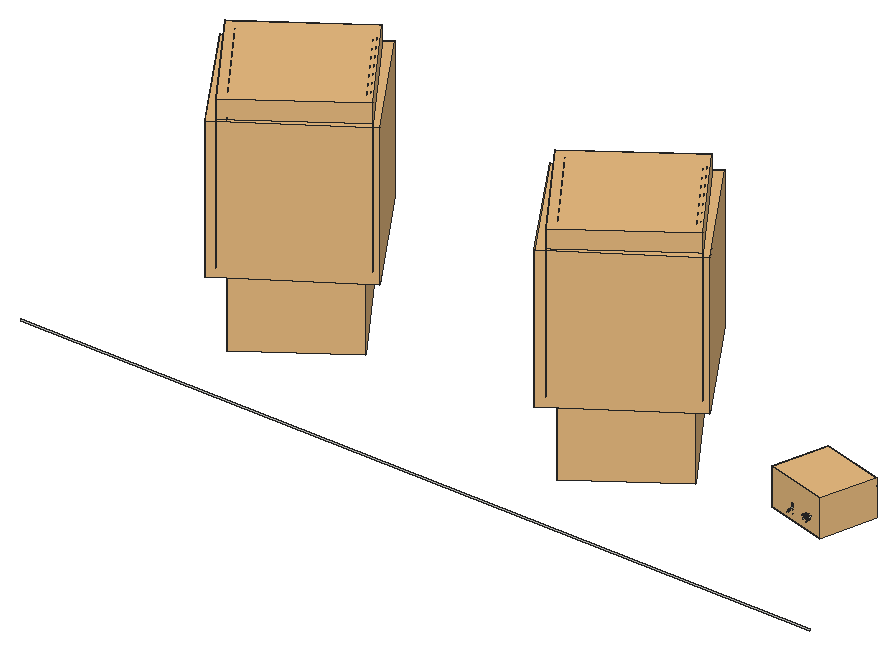
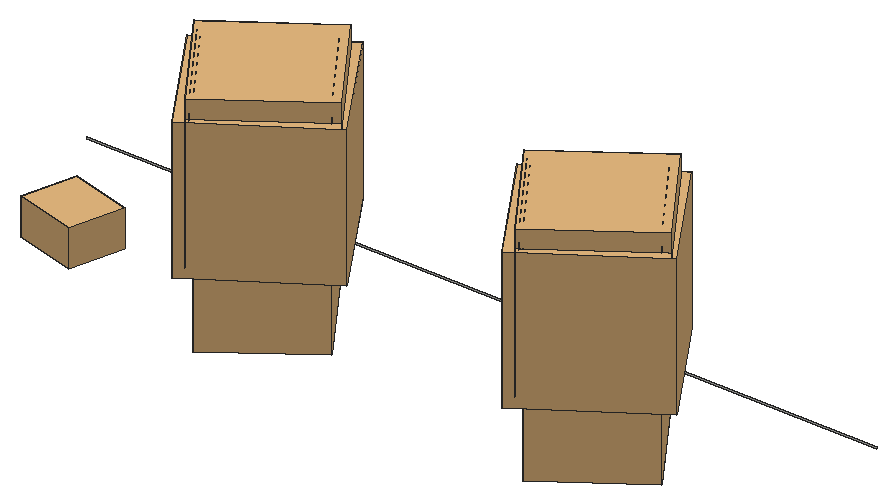
# SketchUp Ruby script. Lengths in inches.
U = 1.inch
M = Sketchup.active_model
def pt(a) = Geom::Point3d.new(a.map { |v| v * U })
def face(e, loops, mat)
  f = e.add_face(loops[0].map { |a| pt(a) })
  loops[1..].each { |l| e.add_face(l.map { |a| pt(a) }).erase! }
  f.material = f.back_material = mat if mat
  f
end
# faces: each face lists its corners as indices into pts; further lists are holes
def faces(e, pts, list, mat = nil) = list.each { |f| face(e, (f[0].is_a?(Array) ? f : [f]).map { |l| l.map { |i| pts[i] } }, mat) }
# xy, xz, yz: faces in a plane at the given z, y or x. An outline is a flat list of corners, or four numbers for a rectangle; further outlines are holes
def ring(l) = l.size == 4 ? [[l[0], l[1]], [l[2], l[1]], [l[2], l[3]], [l[0], l[3]]] : l.each_slice(2).to_a
def flat(e, list, mat, &to3) = list.each { |f| face(e, (f[0].is_a?(Array) ? f : [f]).map { |l| ring(l).map { |u, v| to3.(u, v) } }, mat) }
def xy(e, z, list, mat = nil) = flat(e, list, mat) { |x, y| [x, y, z] }
def xz(e, y, list, mat = nil) = flat(e, list, mat) { |x, z| [x, y, z] }
def yz(e, x, list, mat = nil) = flat(e, list, mat) { |y, z| [x, y, z] }
def lines(e, pts, list) = list.each { |a, b| e.add_line(pt(pts[a]), pt(pts[b])) }
# prism: a flat outline (further loops are holes) pulled along v
def prism(e, loops, v, mat = nil)
  f = face(e, loops, mat); d = Geom::Vector3d.new(v.map { |x| x * U })
  f.pushpull(f.normal.samedirection?(d) ? d.length : -d.length)
end
def box(e, o, s, mat = nil) = prism(e, [[o, [o[0] + s[0], o[1], o[2]], [o[0] + s[0], o[1] + s[1], o[2]], [o[0], o[1] + s[1], o[2]]]], [0, 0, s[2]], mat)
def at(x, y, z, deg = 0) = Geom::Transformation.translation(pt([x, y, z])) * Geom::Transformation.rotation(ORIGIN, Z_AXIS, deg.degrees)
def axes(o, x, y, z) = Geom::Transformation.new([*x, 0, *y, 0, *z, 0, *pt(o).to_a, 1])
def part(name) = M.definitions.add(name)
# library, detail: a bought-in or finely detailed component or shape, given as its bounding box
def library(name, o, s) = part(name).tap { |d| box(d.entities, o, s) }
def detail(e, o, s) = box(e.add_group.entities, o, s)
def put(e, d, t, mat = nil) = e.add_instance(d, t).tap { |i| i.material = mat if mat }
def group(e, t, mat = nil) = e.add_group.tap { |g| g.transformation = t; g.material = mat if mat }.entities
root = M.entities
M.materials.add("028_190k_fullGeometry_Material \#4").color = [120, 148, 64]
M.materials.add("0ad16as01f6asdLeafVar1sfd015as60f1as6").color = [231, 235, 211]
M.materials.add("asdfasdf0165f6asdLeafVar1sfd015as60f1as6").color = [231, 235, 211]
M.materials.add("dw_stemssadfasdfa0sdf1s01d6w1").color = [90, 97, 50]
c1 = library("028_190k_fullGeometry_0",[-319.99,-281.1,-2.15],[577.33,562.38,1159.36])
c2 = library("028_190k_fullGeometry_1",[-333.4,-281.7,421.48],[600.33,578.53,738.83])
c3 = library("028_190k_fullGeometry_2",[-3584003,-3264710,4041818.25],[6566285.5,6460741.75,7903602.75])
c4 = library("028_190k_fullGeometry_3",[-353.86,-324.57,405.22],[652.24,636.69,781.83])
c5 = part("028_190k_fullGeometry_4")
p = [[125.51,152.8,882.93],[125.36,152.82,883.01],[124.8,155.5625,881.05]]
faces(c5.entities,p,[[0,1,2]],"028_190k_fullGeometry_Material \#4")
c6 = part("028_190k_fullGeometry")
g1 = group(c6.entities,at(0,0,0))
put(g1,c1,axes([0,0,0],[0.18998,-0.26642,0],[0.26642,0.18998,0],[0,0,0.32722]))
put(g1,c2,axes([0,0,0],[0.18998,-0.26642,0],[0.26642,0.18998,0],[0,0,0.32722]))
put(g1,c3,axes([0,0,0],[0.00002,-0.00003,0],[0.00003,0.00002,0],[0,0,0.00003]))
put(g1,c4,axes([0,0,0],[0.18998,-0.26642,0],[0.26642,0.18998,0],[0,0,0.32722]))
put(g1,c5,axes([0,0,0],[0.18998,-0.26642,0],[0.26642,0.18998,0],[0,0,0.32722]))
c7 = part("vdw_leaf\#3")
p = [[0,0,0],[-2.77,1.61,2.32],[-4.3125,6.1,4.5],[-3.97,13.49,6.09],[-2.47,18.57,6.3],[-0.2,22.73,5.75],
  [2.54,19.66,6.85],[4.3,15.93,7.09],[5.03,7.6,5.43],[3.32,1.76,2.74]]
faces(c7.entities,p,[[0,1,2,3,4,5],[0,5,6,7,8,9]],"asdfasdf0165f6asdLeafVar1sfd015as60f1as6")
c8 = part("dw_brancj_2\#2")
p = [[9.7,-0.22,29.95],[0.23,-1.96,0.34],[-0.05,1.51,0.11],[9.65,1.51,29.46],[18.64,-8.75,84.43],[18.96,-6.63,84.625],
  [1.53,6.02,63.68],[1.42,8.18,63.25],[-10.58,8.77,161.17],[-10.41,9.98,160.68],[26.34,-9.37,211.72],[26.57,-8.28,211.23]]
faces(c8.entities,p,[[0,1,2],[0,2,3],[4,0,3],[4,3,5],[6,0,3],[6,3,7],[8,6,7],[8,7,9],
  [10,4,5],[10,5,11]],"dw_stemssadfasdfa0sdf1s01d6w1")
c9 = part("vdw_branch2\#3")
put(c9.entities,c7,axes([19.53,-5.9,102.42],[1.12377,-0.50004,0],[0.46097,1.03596,0.47664],[-0.19377,-0.43548,1.13389]))
put(c9.entities,c7,axes([-5.89,6.52,109.44],[-1.07209,0.83679,0],[-0.77141,-0.98832,0.52702],[0.32427,0.41545,1.25373]))
put(c9.entities,c7,axes([-0.44,8.23,75.28],[0.88709,-0.9947,0],[0.92159,0.82189,0.33087],[-0.25219,-0.22491,1.26111]))
put(c9.entities,c7,axes([24.71,-8.97,190.81],[-0.82641,0.91101,0],[-0.83983,-0.76184,0.47664],[0.35303,0.32025,1.13389]))
put(c9.entities,c7,axes([-2.29,8.24,91.35],[1.24603,-0.47303,0],[0.43826,1.15445,0.33087],[-0.11993,-0.31592,1.26111]))
put(c9.entities,c7,axes([12.26,-3.11,37.92],[-0.64625,1.02205,0.22511],[-1.04383,-0.61044,-0.22511],[-0.07533,-0.30931,1.18809]))
put(c9.entities,c7,axes([26.17,-9.17,210.27],[-0.99452,-0.10453,0],[0.09636,-0.91681,0.38752],[-0.04051,0.38539,0.92186]))
put(c9.entities,c7,axes([-6.07,9.4,125.35],[-0.90214,-0.98107,0],[0.90896,-0.83583,0.33087],[-0.24874,0.22873,1.26111]))
put(c9.entities,c7,axes([-4.13,7.29,110.58],[0.44715,-1.078,0.64369],[1.05816,0.63649,0.33087],[-0.58725,0.40856,1.09216]))
put(c9.entities,c7,axes([23.91,-8.22,171.96],[0.62307,0.85009,-0.63406],[-0.71531,0.8798,0.47664],[0.78296,0.12729,0.94004]))
put(c9.entities,c8,at(-0.09,0.18,-0.25),"dw_stemssadfasdfa0sdf1s01d6w1")
put(c9.entities,c7,axes([23.34,-9.65,156.59],[-0.31364,-1.00782,0.58216],[1.10369,-0.17062,0.29925],[-0.17137,0.6239,0.98776]))
put(c9.entities,c7,axes([15.03,-3.37,58.83],[-1.05425,-0.00194,0.58442],[-0.14303,-1.11707,-0.26172],[0.55355,-0.3046,0.99755]))
put(c9.entities,c7,axes([-11.625,9.46,160.37],[0.36812,0.92978,0],[-0.85713,0.33936,0.38752],[0.3603,-0.14265,0.92186]))
put(c9.entities,c7,axes([21.32,-8.53,138.72],[1.21379,0.19904,0],[-0.19904,1.21379,0],[0,0,1.23]))
put(c9.entities,c7,axes([22.54,-9.2,141.43],[-1.02887,0.17955,0.60182],[-0.23387,-1.13057,-0.06253],[0.56696,-0.17376,1.02111]))
put(c9.entities,c7,axes([23.9,-8.82,173.84],[-1.14567,-0.37474,0],[0.35918,-1.0981,0.04438],[-0.01409,0.04308,1.17993]))
put(c9.entities,c7,axes([-7.84,8.92,143.59],[-1.26971,0.40522,0],[-0.37543,-1.17638,0.33087],[0.10274,0.32192,1.26111]))
put(c9.entities,c7,axes([19.77,-8.01,85.98],[-0.32405,-1.14591,0.18674],[1.10278,-0.32969,-0.10948],[0.15845,0.14442,1.16117]))
put(c9.entities,c7,axes([-0.62,5.76,76.34],[-0.08879,1.17576,-0.67771],[-1.34525,-0.16582,-0.11144],[-0.17897,0.66309,1.17383]))
put(c9.entities,c7,axes([20.49,-8.22,121.07],[0.39924,-0.78471,-0.8233],[1.08735,0.33121,0.2116],[0.09035,-0.83005,0.83495]))
put(c9.entities,c7,axes([15.15,-3.72,62.9],[1.16251,0.40128,-0.0211],[-0.39924,1.16074,0.07874],[0.0456,-0.06757,1.2273]))
put(c9.entities,c7,axes([20.72,-8.08,120.26],[-0.03693,1.2277,-0.06551],[-1.22944,-0.03698,0],[-0.00197,0.06548,1.22825]))
put(c9.entities,c7,axes([22.58,-8.36,155.57],[-0.56247,1.09386,0],[-1.00839,-0.51852,0.47664],[0.42389,0.21796,1.13389]))
put(c9.entities,c7,axes([3.97,3.13,57.96],[-1.09459,0.76041,0],[-0.72262,-1.0402,-0.1735],[-0.10109,-0.14552,1.29352]))
put(c9.entities,c7,axes([-10.8,9.06,160.75],[-0.66334,-0.72138,0],[0.66835,-0.61458,0.24329],[-0.1829,0.16818,0.92729]))
put(c9.entities,c7,axes([19.06,-9.3125,103.96],[-1.01345,0.25553,-0.60051],[-0.2265,-1.12952,-0.09839],[-0.59598,0.03076,1.01889]))
put(c9.entities,c7,axes([18.07,-6.2,81.7],[-0.56247,1.09386,0],[-1.00839,-0.51852,0.47664],[0.42389,0.21796,1.13389]))
put(c9.entities,c7,axes([12.95,-0.39,43.31],[0.13044,-1.19832,0],[1.11025,0.12085,0.29925],[-0.30382,-0.03307,1.14057]))
put(c9.entities,c7,axes([2.28,8.28,56.18],[1.32413,-0.31027,0],[0.30923,1.31968,-0.11144],[0.02542,0.1085,1.35543]))
put(c9.entities,c7,axes([-7.55,9.96,143.07],[1.34251,-0.21744,0],[0.20045,1.23761,0.52702],[-0.08426,-0.52024,1.25373]))
put(c9.entities,c7,axes([26.15,-8.25,210.66],[0.94661,-0.25364,0],[0.235,0.87703,0.24329],[-0.06431,-0.24,0.92729]))
put(c9.entities,c7,axes([-6.48,11.37,125.16],[0.64635,1.10315,0.46356],[-1.16569,0.46153,0.52702],[0.27017,-0.6478,1.16488]))
put(c9.entities,c7,axes([25.74,-8.35,191.28],[0.13044,-1.19832,0],[1.11025,0.12085,0.29925],[-0.30382,-0.03307,1.14057]))
put(c9.entities,c7,axes([-5.125,7.47,91.6],[-1.10024,0.63688,0.48318],[-0.78682,-1.00808,-0.46292],[0.14137,-0.65404,1.184]))
c10 = part("vdw_leaf\#1")
p = [[0,0,0],[-2.77,1.61,2.32],[-4.3125,6.1,4.5],[-3.97,13.49,6.09],[-2.47,18.57,6.3],[-0.2,22.73,5.75],
  [2.54,19.66,6.85],[4.3,15.93,7.09],[5.03,7.6,5.43],[3.32,1.76,2.74]]
faces(c10.entities,p,[[0,1,2,3,4,5],[0,5,6,7,8,9]],"0ad16as01f6asdLeafVar1sfd015as60f1as6")
c11 = part("dw_branch_3\#2")
p = [[-10.06,-1.6,62.9],[-0.2,1.54,-0.01],[-10.43,1.54,62.72],[0.18,-1.6,0.17],[-23.75,-21.66,88.91],[-25.7,-20.3,89.55],
  [13.4,11.62,104.56],[13.33,13.52,104.47],[-49.25,-41.87,130.3125],[-50.33,-40.21,130.71],[-4.97,21.13,143.98],[35.61,27.99,178.64],
  [-5.09,23.64,143.96],[35.32,29.14,178.46],[-67.7,-55.38,181.06],[-68.34,-54.45,181.62],[-22.8125,33.9,200.59],[-22.94,35.79,200.41],
  [56.61,36.78,229.75],[56.29,38.09,229.57],[-70.63,-67.46,248.85],[-70.72,-66.33,249.5],[-25.05,43.32,240.75],[-24.98,44.26,240.57]]
faces(c11.entities,p,[[0,1,2],[0,3,1],[4,2,5],[4,0,2],[6,0,2],[6,2,7],[8,4,5],[8,5,9],
  [10,6,7],[11,6,7],[10,7,12],[11,7,13],[14,8,9],[14,9,15],[16,10,12],[16,12,17],
  [18,11,13],[18,13,19],[20,14,15],[20,15,21],[22,16,17],[22,17,23]],"dw_stemssadfasdfa0sdf1s01d6w1")
c12 = part("dw_branch3\#2")
put(c12.entities,c10,axes([-70.33,-63.58,233.32],[-1.00752,0.412,0.78596],[-0.24851,-1.22189,0.32195],[0.83141,0.09817,1.01433]))
put(c12.entities,c10,axes([-66.93,-54.91,182.82],[-0.84976,-0.98359,0.33619],[0.99572,-0.74889,0.32577],[-0.05223,0.46521,1.22907]))
put(c12.entities,c10,axes([-46.12,-39.49,126.35],[1.23843,0.5364,0.23552],[-0.56438,0.94474,0.81599],[0.15707,-0.83465,1.07498]))
put(c12.entities,c10,axes([13.0625,13.13,104.77],[-1.01271,0.69982,-0.26884],[-0.74268,-0.99813,0.19939],[-0.10222,0.31872,1.21473]))
put(c12.entities,c10,axes([-18.87,30.42,186.42],[0.36309,1.06515,-0.56675],[-1.14134,0.49515,0.19939],[0.39128,0.45593,1.10754]))
put(c12.entities,c10,axes([-3.2,4.15,75.77],[-1.04153,0.55414,0.44243],[-0.23365,-1.01045,0.71554],[0.6695,0.50943,0.93801]))
put(c12.entities,c10,axes([23.2,19.41,136.3],[-0.65687,-1.11295,-0.05714],[1.05857,-0.61429,-0.20411],[0.15163,-0.1536,1.24868]))
put(c12.entities,c10,axes([-25.57,35.48,201.32],[-0.64726,0.62827,0.87973],[-0.71635,-1.0172,0.19939],[0.80962,-0.39773,0.87973]))
put(c12.entities,c10,axes([-36.37,-32.14,110.35],[-0.80747,1.09962,0.12544],[-0.83333,-0.50188,-0.96467],[-0.72833,-0.64487,0.96467]))
put(c12.entities,c10,axes([-9.89,26.72,156.79],[0.45529,1.02969,0.56572],[-1.16919,0.33753,0.32662],[0.11537,-0.64297,1.07744]))
put(c12.entities,c10,axes([-26.57,46.1,241.0625],[0.00015,0.80921,0.22536],[-0.83985,0.00446,-0.01542],[-0.01605,-0.22532,0.80906]))
put(c12.entities,c10,axes([-9.2,-2.58,61.06],[-1.10001,-0.40312,0.39014],[0.40883,-1.1116,0.00411],[0.35732,0.13566,1.14763]))
put(c12.entities,c10,axes([-69.91,-63.11,233.93],[1.36249,-0.1432,0],[0.13201,1.25603,0.5309],[-0.05549,-0.52799,1.26295]))
put(c12.entities,c10,axes([32.2,25.46,166.13],[0.06878,-1.29051,-0.05714],[1.22165,0.07415,-0.20411],[0.2113,-0.04403,1.24868]))
put(c12.entities,c10,axes([-5.68,-0.66,44.43],[-0.48448,-1.12287,0.17078],[0.98138,-0.33653,0.57135],[-0.48308,0.36756,1.04626]))
put(c12.entities,c10,axes([43.45,32.81,198.64],[0.5408,1.19584,0.14106],[-0.94242,0.32409,0.86557],[0.74952,-0.45533,0.98656]))
put(c12.entities,c10,axes([12.52,14.14,104.98],[1.02694,0.54888,0.41092],[-0.53566,1.05407,-0.06927],[-0.38969,-0.12321,1.13846]))
put(c12.entities,c10,axes([44.55,32.375,198.73],[-0.65687,-1.11295,-0.05714],[1.05857,-0.61429,-0.20411],[0.15163,-0.1536,1.24868]))
put(c12.entities,c10,axes([-5.67,21.17,141.44],[-1.10726,0.43603,-0.32953],[-0.49537,-1.03435,0.29588],[-0.17521,0.40597,1.12589]))
put(c12.entities,c10,axes([55.69,37.84,229.48],[0.18984,0.96334,0.18958],[-0.71996,0.0053,0.69399],[0.66755,-0.26823,0.69457]))
put(c12.entities,c10,axes([-21.52,36.85,205.2],[0.72606,-0.98817,0.14519],[0.94364,0.7084,0.10251],[-0.16885,0.05176,1.19664]))
put(c12.entities,c10,axes([-68.51,-56.35,196.07],[1.16319,0.72381,0],[-0.66725,1.0723,0.5309],[0.28049,-0.45075,1.26295]))
put(c12.entities,c11,at(0.01,-0.09,-0.02),"dw_stemssadfasdfa0sdf1s01d6w1")
put(c12.entities,c10,axes([-2.49,5.18,75.91],[0.78614,-0.90346,-0.30078],[0.86953,0.79562,-0.11715],[0.28546,-0.14014,1.16705]))
put(c12.entities,c10,axes([-23.125,-16.22,82.25],[0.32175,1.32576,0.12544],[-1.33153,0.31835,0.05068],[0.01989,-0.13382,1.3633]))
put(c12.entities,c10,axes([-23.75,41.99,230.3],[0.85958,-0.87451,0.14519],[0.66531,0.75721,0.62192],[-0.54076,-0.36226,1.01955]))
put(c12.entities,c10,axes([27.07,22.48,149.34],[0.92952,-0.64745,-0.62467],[0.50188,1.074,-0.36637],[0.71693,0.02135,1.04468]))
put(c12.entities,c10,axes([17.66,16.25,119.93],[-0.91649,0.83891,-0.3601],[-0.87434,-0.77966,0.40896],[0.0492,0.54447,1.14321]))
put(c12.entities,c10,axes([-68.37,-54.54,181.63],[0.32047,1.28399,0.35434],[-1.33153,0.31835,0.05068],[-0.03484,-0.35624,1.32241]))
put(c12.entities,c10,axes([-28.98,-27.1,96.48],[-0.8814,-0.35966,-0.98523],[0.75246,-1.11336,-0.26672],[-0.73065,-0.71272,0.91382]))
put(c12.entities,c10,axes([-15.23,28.43,172.72],[-1.21149,0.11898,0.32517],[-0.09739,-1.25259,0.09551],[0.33228,0.0667,1.21356]))
put(c12.entities,c10,axes([-17.5625,31.23,186.85],[-0.49275,-1.12287,0.14519],[0.95014,-0.33653,0.62192],[-0.53717,0.36756,1.01955]))
put(c12.entities,c10,axes([26.7,21.22,149.39],[-1.00104,0.22334,0.83093],[0.36894,-1.0402,0.72406],[0.77731,0.78134,0.72643]))
put(c12.entities,c10,axes([-31.125,-24.87,97.38],[0.75482,-0.86936,0.69068],[-0.00159,0.80023,1.00899],[-1.08766,-0.58016,0.45842]))
put(c12.entities,c10,axes([-71.21,-66.73,248.67],[0.25207,0.96771,0],[-0.8921,0.23237,0.38752],[0.375,-0.09768,0.92186]))
put(c12.entities,c10,axes([-24.11,41.05,229.55],[-1.11612,0.51924,-0.26884],[-0.56394,-1.10897,0.19939],[-0.15444,0.29694,1.21473]))
put(c12.entities,c10,axes([6.75,8.37,91.63],[-0.33418,-1.12287,0.39014],[1.13558,-0.33653,0.00411],[0.10478,0.36756,1.14763]))
put(c12.entities,c10,axes([-26,45.89,241.63],[-0.26986,-0.70824,-0.32129],[0.56818,-0.39091,0.38449],[-0.49365,-0.09775,0.63011]))
put(c12.entities,c10,axes([3.74,17.32,124.35],[0.22441,1.22913,-0.16274],[-1.07812,0.11178,-0.64246],[-0.61228,0.25367,1.07162]))
put(c12.entities,c10,axes([-5.44,22.27,140.88],[1.2203,0.00475,0.31374],[-0.097,1.20386,0.35905],[-0.29841,-0.37189,1.1663]))
put(c12.entities,c10,axes([-13.79,29.35,173.31],[0.83169,-0.90108,0.14519],[0.68877,0.73594,0.62192],[-0.55187,-0.34509,1.01955]))
put(c12.entities,c10,axes([-16.92,-7.26,72.98],[1.30647,0.30378,-0.27886],[0.07026,0.74892,1.14503],[0.40633,-1.10623,0.69861]))
put(c12.entities,c10,axes([4.8,17.55,125.22],[-0.25598,-1.17842,0.26559],[1.01553,-0.08455,0.60363],[-0.56975,0.35087,1.00767]))
put(c12.entities,c10,axes([5.3125,8.35,91.45],[0.00638,1.22913,-0.27714],[-1.16413,0.11178,0.46895],[0.48205,0.25367,1.13617]))
put(c12.entities,c10,axes([38.12,30.57,183.07],[1.12534,0.26182,-0.63833],[-0.46674,1.18829,-0.33545],[0.5081,0.51169,1.10563]))
put(c12.entities,c10,axes([-70.41,-60.38,214.47],[-0.41425,1.30587,0],[-1.20383,-0.38188,0.5309],[0.50605,0.16053,1.26295]))
put(c12.entities,c10,axes([37.03,28.75,180.67],[-1.12533,0.00102,-0.63799],[-0.00113,-1.2408,0],[-0.62497,0.00057,1.10237]))
put(c12.entities,c10,axes([30.71,25.35,165.96],[-0.1364,1.29314,0.22715],[-1.08768,-0.23921,0.70862],[0.73536,-0.11394,1.09026]))
put(c12.entities,c10,axes([-38.05,-30.84,110.67],[-0.31533,-1.27379,-0.2839],[1.018,-0.40311,0.67794],[-0.74394,-0.05723,1.08307]))
put(c12.entities,c10,axes([50.11,34.45,213.36],[-1.05669,0.74401,-0.05714],[-0.616,-0.82138,0.69675],[0.37221,0.60904,1.04705]))
put(c12.entities,c10,axes([-65.32,-58.78,200.07],[-1.14597,-0.19668,-0.6713],[0.21784,-1.26924,0],[-0.64812,-0.11124,1.139]))
put(c12.entities,c10,axes([-53.2,-43.37,143.59],[-0.72817,-1.09167,-0.2839],[0.82127,-0.72411,0.67794],[-0.71934,0.19815,1.08307]))
put(c12.entities,c10,axes([-61.1,-50.25,163.67],[-0.52887,1.19686,-0.30066],[-1.10762,-0.57104,-0.32484],[-0.42634,0.12264,1.23812]))
put(c12.entities,c10,axes([-54.12,-42.96,142.67],[0.32175,1.32576,0.12544],[-1.33153,0.31835,0.05068],[0.01989,-0.13382,1.3633]))
put(c12.entities,c10,axes([22.03,20.08,132.3],[1.17066,0.5058,-0.34078],[-0.35758,1.16671,0.50333],[0.49407,-0.35407,1.17172]))
put(c12.entities,c10,axes([-8.59,26.04,158.21],[-0.49275,-1.12287,0.14519],[0.95014,-0.33653,0.62192],[-0.53717,0.36756,1.01955]))
put(c12.entities,c10,axes([49.92,34.03,213.7],[1.24742,-0.35176,0.25024],[0.42127,1.159,-0.4708],[-0.09426,0.52477,1.20753]))
put(c12.entities,c10,axes([-70.34,-67.02,249.05],[-0.57048,-0.79684,0],[0.73827,-0.52855,0.24329],[-0.20203,0.14464,0.92729]))
put(c12.entities,c10,axes([56.04,36.81,228.63],[0.33451,-0.90845,-0.15237],[0.87636,0.33365,-0.06538],[0.11487,-0.11636,0.94597]))
put(c12.entities,c10,axes([-69.93,-60.58,214.88],[-0.45293,-0.99272,-0.78227],[1.14635,-0.58199,0.07483],[-0.40282,-0.65636,1.06615]))
put(c12.entities,c10,axes([-16.77,-8.59,72.7],[-1.22785,0.11509,0.53076],[-0.24879,-1.22495,-0.30991],[0.46742,-0.38989,1.16587]))
put(c12.entities,c10,axes([18.29,17.18,119.24],[1.19981,-0.45946,0.3029],[0.40159,1.22775,0.27158],[-0.37626,-0.1547,1.25575]))
put(c12.entities,c10,axes([-6.73,-0.68,43.74],[0.05346,1.22913,-0.27201],[-1.22696,0.11178,0.26396],[0.28163,0.25367,1.20164]))
put(c12.entities,c10,axes([-58.57,-48.42,160.98],[0.43385,-1.23789,0.39533],[1.04879,0.57965,0.66404],[-0.76727,0.09236,1.13122]))
put(c12.entities,c10,axes([-23.4,38.49,215.38],[0.06762,1.22913,-0.26884],[-1.23909,0.11178,0.19939],[0.21835,0.25367,1.21473]))
put(c12.entities,c10,axes([-22.21,-16.62,83.17],[-0.72817,-1.09167,-0.2839],[0.82127,-0.72411,0.67794],[-0.71934,0.19815,1.08307]))
put(c12.entities,c10,axes([-45.7,-40.77,126.53],[-1.33715,-0.0713,-0.0976],[0.07167,-1.28508,-0.04314],[-0.09306,-0.0492,1.31098]))
put(c12.entities,c10,axes([-22.39,38.51,216.12],[-0.49275,-1.12287,0.14519],[0.95014,-0.33653,0.62192],[-0.53717,0.36756,1.01955]))
c13 = part("vdw_leaf\#2")
p = [[0,0,0],[-2.77,1.61,2.32],[-4.3125,6.1,4.5],[-3.97,13.49,6.09],[-2.47,18.57,6.3],[-0.2,22.73,5.75],
  [2.54,19.66,6.85],[4.3,15.93,7.09],[5.03,7.6,5.43],[3.32,1.76,2.74]]
faces(c13.entities,p,[[0,1,2,3,4,5],[0,5,6,7,8,9]],"asdfasdf0165f6asdLeafVar1sfd015as60f1as6")
c14 = part("dg_branch_1\#2")
p = [[46.12,1.57,35.62],[46,5.42,35.41],[0.14,1.79,0.05],[0.26,-2.0625,0.27],[74.05,2.99,75.8],[74.11,5.28,75.58],
  [103.46,0.47,94.74],[104.03,2.92,94.84],[81.14,16.92,120.46],[81.2,18.78,120.24],[130.47,-5.6875,130.27],[130.58,-3.66,129.85],
  [80.82,34.4375,191.22],[80.64,35.93,190.9],[148.49,-14.56,203.24],[148.9,-12.8125,203.11],[81.08,37.95,226.93],[81.4,39.1,227.03],
  [157.45,-18.19,250.77],[157.7,-17.01,250.41]]
faces(c14.entities,p,[[0,1,2,3],[4,0,1],[4,1,5],[6,4,5],[6,5,7],[8,4,5],[8,5,9],[10,6,7],
  [10,7,11],[12,8,9],[12,9,13],[14,10,11],[14,11,15],[16,12,13],[16,13,17],[18,14,15],
  [18,15,19]],"dw_stemssadfasdfa0sdf1s01d6w1")
c15 = part("vdw_branch1\#3")
put(c15.entities,c13,axes([120.69,-2.42,117.31],[1.12221,-0.24063,-0.65809],[0.19207,1.24776,-0.12871],[0.65778,0.01392,1.11658]))
put(c15.entities,c13,axes([81,38.9,226.05],[0.7888,-0.58155,0],[0.48308,0.65523,0.47],[-0.28484,-0.38635,0.83138]))
put(c15.entities,c13,axes([78.08,12.69,106.05],[-1.43826,-0.02353,-0.03177],[0.0088,-1.31777,0.57755],[-0.03854,0.57714,1.31741]))
put(c15.entities,c13,axes([130.18,-4.73,130.41],[-0.38031,-1.29044,-0.11242],[1.20662,-0.31032,-0.51987],[0.47109,-0.24694,1.24081]))
put(c15.entities,c13,axes([157.08,-17.89,249.93],[-0.91355,0.40674,0],[-0.37496,-0.84216,0.38752],[0.15762,0.35401,0.92186]))
put(c15.entities,c13,axes([90.64,3.03,86.49],[0.32514,-0.85045,-0.99675],[0.69523,0.98247,-0.61148],[1.11061,-0.36604,0.67459]))
put(c15.entities,c13,axes([80.15,28.42,160.95],[-0.16039,0.95636,-1.06292],[-1.41646,0.03966,0.24943],[0.19509,1.07422,0.93709]))
put(c15.entities,c13,axes([126.74,-5.45,129.22],[-0.59819,0.96152,-0.6841],[-0.85772,0.12575,0.92675],[0.75427,0.88089,0.57856]))
put(c15.entities,c13,axes([133.22,-6.12,150.66],[-0.93823,0.76985,0.59124],[-0.47726,-1.08188,0.65135],[0.84525,0.24366,1.02405]))
put(c15.entities,c13,axes([80.43,22.89,141.32],[-1.42571,-0.19312,0.01373],[0.18338,-1.31425,0.5561],[-0.0621,0.5528,1.32692]))
put(c15.entities,c13,axes([33.14,0.88,26.42],[-0.13338,1.31536,0.04876],[-1.04528,-0.13221,0.7073],[0.72315,0.03348,1.07497]))
put(c15.entities,c13,axes([152.63,-15.08,221.76],[-1.28188,0.41945,0.0579],[-0.3638,-1.18547,0.53367],[0.21665,0.49113,1.23869]))
put(c15.entities,c13,axes([80.05,28.28,160.33],[-0.46732,-1.26661,0.40679],[1.27397,-0.40257,0.21004],[-0.07408,0.44645,1.30501]))
put(c15.entities,c13,axes([153.95,-14.8,235.875],[0.39005,1.07743,0.20605],[-0.96443,0.25296,0.50293],[0.42961,-0.3464,0.99807]))
put(c15.entities,c13,axes([80.2,24.22,141.74],[1.33062,-0.46576,0.02628],[0.44746,1.2746,-0.06608],[-0.00197,0.0722,1.37936]))
put(c15.entities,c13,axes([145.48,-12.5,188.92],[-1.32952,0.16983,0.16138],[-0.09299,-1.2361,0.53471],[0.21503,0.51548,1.22904]))
put(c15.entities,c13,axes([139.64,-9.18,171.24],[0.05682,1.30088,0.23414],[-1.13176,-0.05343,0.57151],[0.58357,-0.22963,1.13417]))
put(c15.entities,c13,axes([70.95,4.35,71.98],[-1.1081,-0.41873,0.64752],[0.33675,-1.28259,-0.25313],[0.6937,-0.04625,1.15721]))
put(c15.entities,c13,axes([59.85,4.55,56.17],[-0.26797,1.24526,0.35754],[-0.9369,-0.41634,0.74783],[0.83377,-0.10389,0.98674]))
put(c15.entities,c13,axes([33.11,3.36,25.66],[-0.57817,-1.07968,-0.5679],[1.11554,-0.21356,-0.7297],[0.49375,-0.78178,0.98363]))
put(c15.entities,c14,at(-0.21,0.34,-0.17),"dw_stemssadfasdfa0sdf1s01d6w1")
put(c15.entities,c13,axes([80.91,19.01,122.53],[-0.84258,1.13222,-0.27981],[-1.15093,-0.75138,0.42537],[0.18861,0.47293,1.3457]))
put(c15.entities,c13,axes([119.8,-1.22,114.1],[-1.3235,-0.25012,0.09101],[0.25933,-1.31572,0.15537],[0.05991,0.1698,1.33794]))
put(c15.entities,c13,axes([46.29,5.1,38.04],[0.98937,0.73827,-0.47585],[-0.72359,1.03721,0.10473],[0.44068,0.18581,1.20453]))
put(c15.entities,c13,axes([81.1875,33.03,184.45],[1.33883,0.26986,0.35053],[-0.09581,1.22087,-0.57399],[-0.42216,0.53228,1.20262]))
put(c15.entities,c13,axes([80.16,36.28,206.98],[-0.83993,0.85737,-0.6234],[-1.05964,-0.65701,0.5241],[0.02941,0.81391,1.07976]))
put(c15.entities,c13,axes([154.86,-16.15,234.87],[0.02509,-1.15302,-0.28506],[1.1487,-0.04894,0.29908],[-0.30202,-0.28195,1.11384]))
put(c15.entities,c13,axes([108.77,-0.33,101.14],[-0.47691,-1.03266,-0.72709],[1.25395,-0.29455,-0.40416],[0.15052,-0.81814,1.06325]))
put(c15.entities,c13,axes([89.79,3.01,85.87],[-0.61344,0.75518,0.8965],[-0.17758,-1.01824,0.73622],[1.13385,0.22574,0.58569]))
put(c15.entities,c13,axes([81.56,20.31,123.29],[0.37259,-1.3435,0.21057],[1.29385,0.32364,-0.22445],[0.16906,0.25791,1.34638]))
put(c15.entities,c13,axes([46.45,1.82,36.74],[-0.77883,0.29892,1.0614],[0.19124,-1.24314,0.49044],[1.08598,0.43329,0.67484]))
put(c15.entities,c13,axes([71.37,4.02,72.32],[0.72905,0.81546,-0.74421],[-0.66805,0.98958,0.42988],[0.8391,0.14186,0.97745]))
put(c15.entities,c13,axes([136.59,-5.88,150.53],[0.85845,-0.99897,-0.12437],[0.96526,0.81273,0.13453],[-0.02572,-0.18182,1.28292]))
put(c15.entities,c13,axes([80.375,38.8,225.86],[-0.25178,0.96778,0],[-0.89216,-0.23211,0.38752],[0.37503,0.09757,0.92186]))
put(c15.entities,c13,axes([74.43,7.99,85.38],[-1.05703,0.91669,-0.33543],[-0.95806,-0.87958,0.61531],[0.18697,0.6754,1.25659]))
put(c15.entities,c13,axes([76.57,9.74,89.32],[0.63146,-1.21538,0.33508],[1.18148,0.49387,-0.43517],[0.26321,0.48577,1.26593]))
put(c15.entities,c13,axes([81.6875,36.97,207.4],[0.09422,-1.04424,0.38486],[1.01646,0.1939,0.27727],[-0.33299,0.33382,0.98727]))
put(c15.entities,c13,axes([157.29,-17.17,249.98],[0.50586,-0.50586,0],[0.38853,0.38853,0.41105],[-0.29684,-0.29684,0.56115]))
put(c15.entities,c13,axes([79.92,15.8,106.09],[1.03917,-0.29343,-0.90675],[-0.14587,1.22131,-0.5624],[0.92163,0.5191,0.88824]))
put(c15.entities,c13,axes([61.95,3.88,56.26],[0.41243,-1.28546,0],[1.17466,0.37688,-0.54831],[0.5221,0.16751,1.23363]))
put(c15.entities,c13,axes([151.99,-14.79,208.15],[-0.48571,-1.21723,-0.32393],[1.25386,-0.50033,0],[-0.12005,-0.30087,1.31056]))
put(c15.entities,c13,axes([108.44,0.62,102.22],[0.82183,0.96078,0.38967],[-0.62327,0.08618,1.10203],[0.79141,-0.88661,0.51693]))
put(c15.entities,c13,axes([145.6,-10.56,188.62],[1.03241,-0.02554,-0.82693],[0.3944,1.11584,0.45794],[0.70325,-0.61672,0.89706]))
put(c15.entities,c13,axes([78.59,32.3,183.89],[-1.12675,-0.42036,0.43987],[0.5899,-0.98149,0.57312],[0.14901,0.70693,1.05726]))
put(c15.entities,c13,axes([152.08,-13.42,223.37],[0.79993,-0.44251,-0.69938],[0.68456,0.82615,0.26026],[0.41048,-0.60953,0.85515]))
put(c15.entities,c13,axes([140.71,-8.74,170.55],[0.41903,-1.24177,-0.32393],[1.26224,0.33728,0.33986],[-0.23168,-0.40836,1.26573]))
put(c15.entities,c13,axes([149.25,-12.53,205.78],[1.24456,0.38285,0.23414],[-0.42999,1.04826,0.57151],[-0.02056,-0.62679,1.13417]))
c16 = library("Broadleaf plant",[0,0,0],[62.33,72.62,41.59])
xz(root,0,[[0,-9,1338.625,-6]])
put(root,c6,at(293.26,225.89,-5.3))
put(root,c6,at(852.51,225.89,-5.3))
put(root,c9,axes([1132.92,249.53,-3.44],[-0.06851,-0.04024,-0.04853],[0.04493,-0.07649,0],[-0.03401,-0.01998,0.09777]))
put(root,c12,axes([1137.74,248.73,-5.91],[-0.0835,0.03705,-0.03198],[-0.01833,-0.07755,-0.06358],[-0.04138,-0.04041,0.09269]))
put(root,c12,axes([1135.98,248.31,-3.51],[0.11088,0,0],[0,0.11088,0],[0,0,0.13644]))
put(root,c15,axes([1145.27,220.56,-3.7],[-0.07583,0.05409,0],[-0.05409,-0.07583,0],[0,0,0.11461]))
put(root,c15,axes([1135.67,248.46,-3.7],[0.01294,-0.09448,0],[0.09448,0.01294,0],[0,0,0.11734]))
put(root,c9,axes([1143.21,219.7,-3.44],[-0.06851,-0.04024,-0.04853],[0.04493,-0.07649,0],[-0.03401,-0.01998,0.09777]))
put(root,c9,axes([1143.12,220.61,-2.94],[-0.10632,-0.02382,-0.02533],[0.02424,-0.1082,0],[-0.02009,-0.0045,0.13407]))
put(root,c12,axes([1147.22,223.25,-1.4],[0.06434,-0.05829,0.02833],[0.05722,0.06809,0.01535],[-0.02555,0.00573,0.10572]))
put(root,c9,axes([1137.35,248.41,-4.91],[0.06689,-0.0646,-0.07431],[0.07703,0.07976,0],[0.04344,-0.04195,0.11443]))
put(root,c12,axes([1148.03,218.9,-5.91],[-0.0835,0.03705,-0.03198],[-0.01833,-0.07755,-0.06358],[-0.04138,-0.04041,0.09269]))
put(root,c12,axes([1146.27,218.48,-3.51],[0.11088,0,0],[0,0.11088,0],[0,0,0.13644]))
put(root,c9,axes([1147.79,221.93,-4.3],[0.00659,0.0958,-0.06822],[-0.11062,0.0076,0],[0.0038,0.05531,0.11816]))
put(root,c15,axes([1145.96,218.63,-3.7],[0.01294,-0.09448,0],[0.09448,0.01294,0],[0,0,0.11734]))
put(root,c9,axes([1150.58,219.33,-4.8],[0.01852,0.08442,-0.0614],[-0.09748,0.02138,0],[0.01069,0.04874,0.10635]))
put(root,c9,axes([1147.65,218.58,-4.91],[0.06689,-0.0646,-0.07431],[0.07703,0.07976,0],[0.04344,-0.04195,0.11443]))
put(root,c9,axes([1151.2,218.875,-2.94],[0.10716,0.01972,-0.02533],[-0.02007,0.10905,0],[0.02025,0.00373,0.13407]))
put(root,c15,axes([1149.68,219.83,-3.7],[0.07973,0.03352,0],[-0.03352,0.07973,0],[0,0,0.10642]))
put(root,c16,axes([1205.88,187.17,1.89],[0.38318,1.43005,0],[-1.43005,0.38318,0],[0,0,1.4805]))
put(root,c15,axes([1190.17,211.61,0.51],[-0.11174,0.0797,0],[-0.0797,-0.11174,0],[0,0,0.16889]))
put(root,c9,axes([1187.13,210.35,0.89],[-0.10096,-0.0593,-0.07152],[0.0662,-0.11272,0],[-0.05012,-0.02944,0.14408]))
put(root,c9,axes([1186.99,211.69,1.63],[-0.15667,-0.0351,-0.03733],[0.03572,-0.15945,0],[-0.0296,-0.00663,0.19757]))
put(root,c12,axes([1193.04,215.58,3.91],[0.09481,-0.08589,0.04174],[0.08433,0.10034,0.02262],[-0.03765,0.00844,0.15579]))
put(root,c12,axes([1194.24,209.17,-2.75],[-0.12304,0.0546,-0.04713],[-0.02701,-0.11428,-0.0937],[-0.06098,-0.05955,0.13659]))
